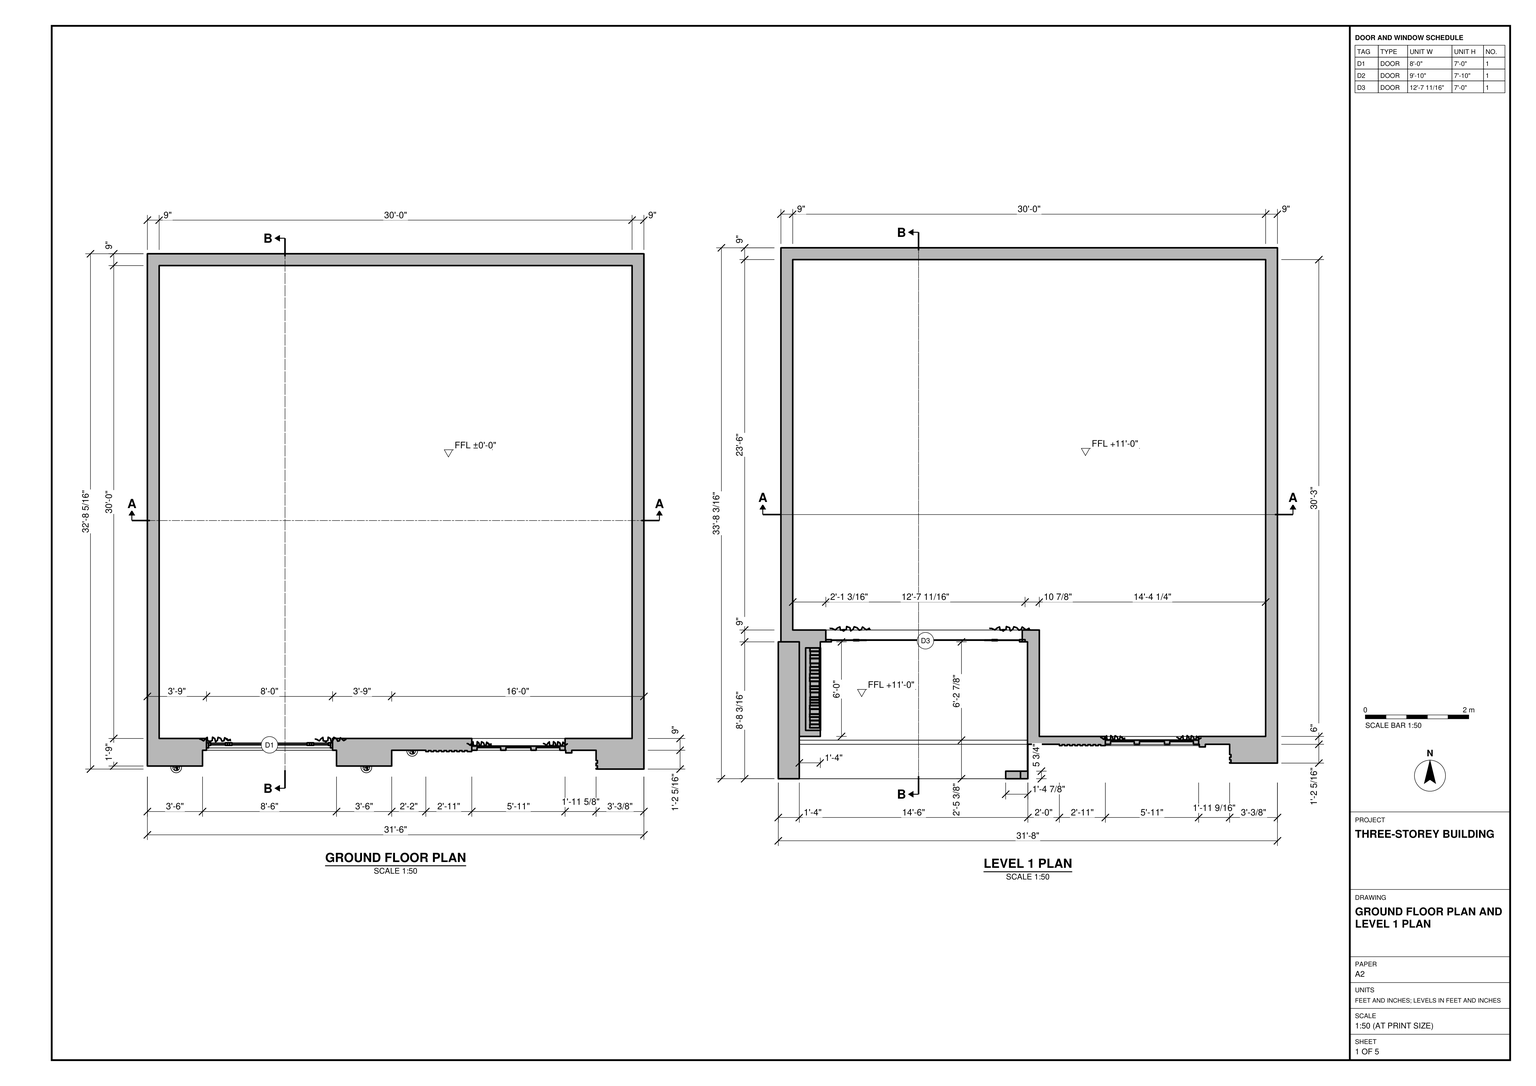
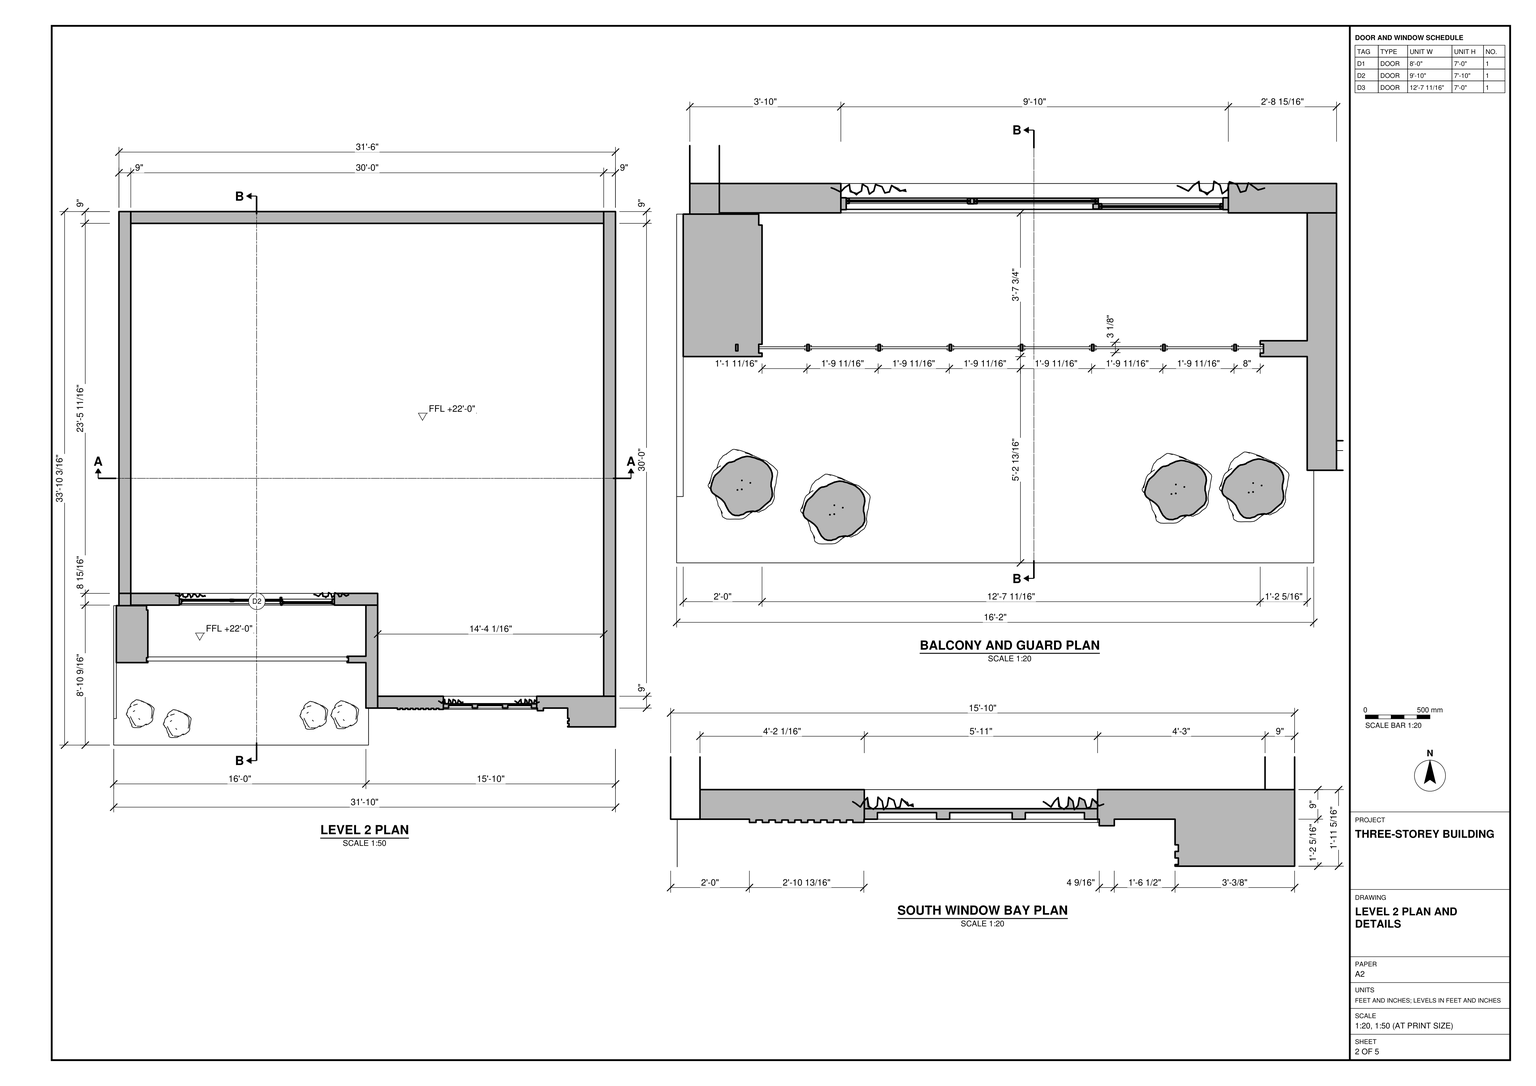
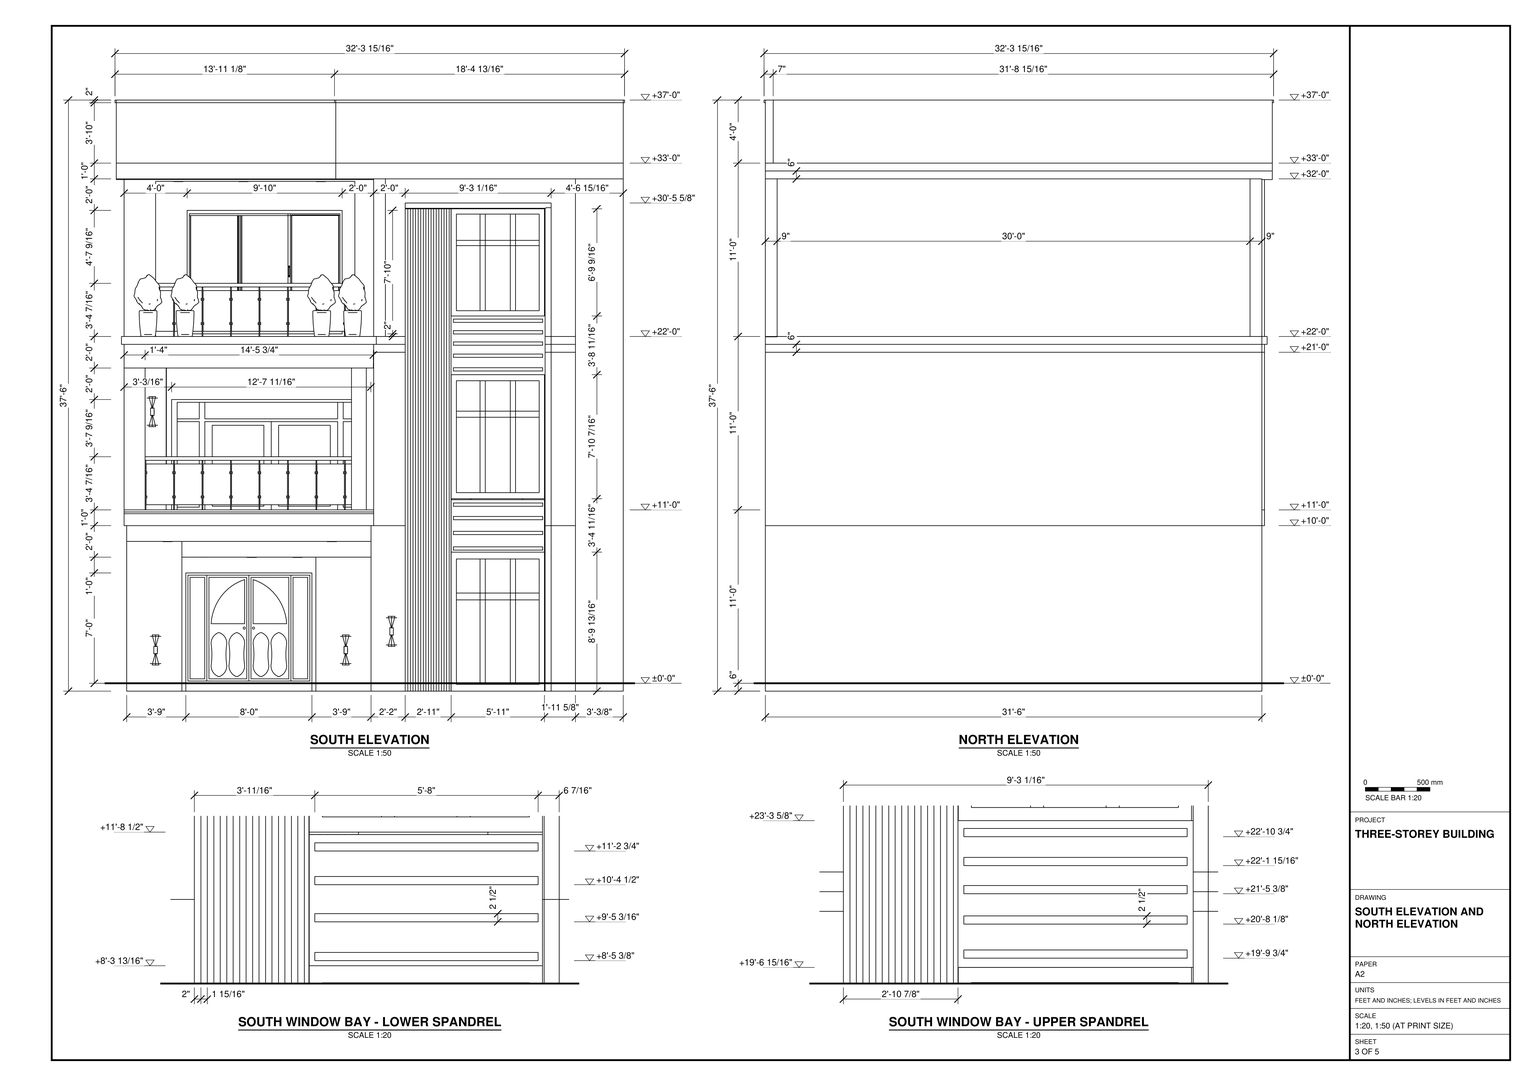
Build the three-storey building in SketchUp from task_files/diagram_01.pdf. Work in feet and inches. Orient the entrance to the south as drawn. The overall dimensions, including projections, are 32'-3 15/16" across the south elevation, 33'-10 3/16" from front to back and 37'-6" from base to top. Set the finished floor levels at ±0'-0", +11'-0" and +22'-0".

Use the floor plans to lay out the 9" perimeter walls and the changes in wall thickness and alignment at the south facade. Keep the main floor areas open as drawn. Model the base, floor slabs and flat roof with its parapet. On the left of the south elevation, place the double entrance with sidelights below the two balconies. Set the balcony doors back behind the glass guards, and extend the upper balcony slab beyond its guard as shown in the balcony plan. On the right, align the divided windows vertically. Model the ribbed strip beside the glazing and the horizontal bands between windows, using the enlarged spandrel details. Keep the north elevation plain apart from the slab and roof lines.

Place the potted plants on the upper balcony and wall lights where drawn. Decor and loose items may be any suitable library components. Keep shell elements such as walls, slabs and roof, and each furniture or joinery piece, in separate groups or components; use components for repeated parts. Save one SketchUp model as output_files/three_storey_building_with_balconies_and_window_bay.skp.

# SketchUp Ruby script. Lengths in inches.
U = 1.inch
M = Sketchup.active_model
def pt(a) = Geom::Point3d.new(a.map { |v| v * U })
def face(e, loops, mat)
  f = e.add_face(loops[0].map { |a| pt(a) })
  loops[1..].each { |l| e.add_face(l.map { |a| pt(a) }).erase! }
  f.material = f.back_material = mat if mat
  f
end
# faces: each face lists its corners as indices into pts; further lists are holes
def faces(e, pts, list, mat = nil) = list.each { |f| face(e, (f[0].is_a?(Array) ? f : [f]).map { |l| l.map { |i| pts[i] } }, mat) }
# xy, xz, yz: faces in a plane at the given z, y or x. An outline is a flat list of corners, or four numbers for a rectangle; further outlines are holes
def ring(l) = l.size == 4 ? [[l[0], l[1]], [l[2], l[1]], [l[2], l[3]], [l[0], l[3]]] : l.each_slice(2).to_a
def flat(e, list, mat, &to3) = list.each { |f| face(e, (f[0].is_a?(Array) ? f : [f]).map { |l| ring(l).map { |u, v| to3.(u, v) } }, mat) }
def xy(e, z, list, mat = nil) = flat(e, list, mat) { |x, y| [x, y, z] }
def xz(e, y, list, mat = nil) = flat(e, list, mat) { |x, z| [x, y, z] }
def yz(e, x, list, mat = nil) = flat(e, list, mat) { |y, z| [x, y, z] }
def lines(e, pts, list) = list.each { |a, b| e.add_line(pt(pts[a]), pt(pts[b])) }
# prism: a flat outline (further loops are holes) pulled along v
def prism(e, loops, v, mat = nil)
  f = face(e, loops, mat); d = Geom::Vector3d.new(v.map { |x| x * U })
  f.pushpull(f.normal.samedirection?(d) ? d.length : -d.length)
end
def box(e, o, s, mat = nil) = prism(e, [[o, [o[0] + s[0], o[1], o[2]], [o[0] + s[0], o[1] + s[1], o[2]], [o[0], o[1] + s[1], o[2]]]], [0, 0, s[2]], mat)
def at(x, y, z, deg = 0) = Geom::Transformation.translation(pt([x, y, z])) * Geom::Transformation.rotation(ORIGIN, Z_AXIS, deg.degrees)
def axes(o, x, y, z) = Geom::Transformation.new([*x, 0, *y, 0, *z, 0, *pt(o).to_a, 1])
def part(name) = M.definitions.add(name)
# library, detail: a bought-in or finely detailed component or shape, given as its bounding box
def library(name, o, s) = part(name).tap { |d| box(d.entities, o, s) }
def detail(e, o, s) = box(e.add_group.entities, o, s)
def put(e, d, t, mat = nil) = e.add_instance(d, t).tap { |i| i.material = mat if mat }
def group(e, t, mat = nil) = e.add_group.tap { |g| g.transformation = t; g.material = mat if mat }.entities
root = M.entities
M.materials.add("Emissive").color = [231, 236, 189]
M.materials["Emissive"].alpha = 1
M.materials.add("Glass Window Turquoise Blue").color = [210, 210, 210]
M.materials["Glass Window Turquoise Blue"].alpha = 0.25
M.materials.add("[0131_Silver]").color = [28, 28, 28]
M.materials.add("[Color A08]").color = [102, 0, 0]
M.materials.add("[Color M06]").color = [86, 86, 86]
M.materials.add("[Color M07]").color = [58, 58, 58]
M.materials.add("[Translucent_Glass_Blue]1").color = [255, 255, 255]
M.materials["[Translucent_Glass_Blue]1"].alpha = 0
M.materials.add("[Wood Cherry Original]").color = [152, 86, 42]
c1 = library("storefront door with transom",[0.96,31.97,0],[7.26,76.03,84.48])
c2 = library("Double Doors",[0,0,0],[118.11,4.72,98.43])
c3 = library("Sliding-door-2700x2100x89",[-27.94,-98.64,-16.57],[106.3,5.83,82.68])
c4 = library("Curtains 004",[-15.59,-2.26,0],[31.18,4.52,116.91])
c5 = library("Books  43-02",[-15.21,-3.875,0],[30.42,7.76,10.71])
c6 = library("Books and Flasks 103-12",[-7.1,-3.71,0],[14.22,7.42,6.38])
c7 = part("Group\#11")
xy(c7.entities,0,[[0,0,0.39,2.125]],"[0131_Silver]")
xy(c7.entities,1.5,[[0,0,0.39,2.125]],"[0131_Silver]")
xz(c7.entities,0,[[0,0,0.39,1.5]],"[0131_Silver]")
xz(c7.entities,2.125,[[0,0,0.39,1.5]],"[0131_Silver]")
yz(c7.entities,0,[[0,0,2.125,1.5]],"[0131_Silver]")
yz(c7.entities,0.39,[[0,0,2.125,1.5]],"[0131_Silver]")
c8 = part("Glass railing panel")
xy(c8.entities,0,[[-0.59,0,0,63.98]])
xy(c8.entities,37.71,[[-0.59,0,0,63.98]])
xz(c8.entities,0,[[-0.59,0,0,37.71]])
xz(c8.entities,63.98,[[-0.59,0,0,37.71]])
yz(c8.entities,-0.59,[[0,0,63.98,37.71]])
yz(c8.entities,0,[[0,0,63.98,0,63.98,37.71,0,37.71,0,30.53,1.75,30.53,1.75,28.71,0,28.71],[-0.4,28.71,0,30.53],[0,28.71,1.75,30.53]])
p = [[0,63.98,30.53],[0.39,63.98,30.53]]
lines(c8.entities,p,[[0,1]])
put(c8.entities,c7,axes([0,62.22,28.71],[1,0,0],[0,1.01246,0],[0,0,1.2158]))
put(c8.entities,c7,axes([0,62.22,6.27],[1,0,0],[0,1.01246,0],[0,0,1.2158]))
put(c8.entities,c7,axes([0,0.6,28.71],[1,0,0],[0,1.01246,0],[0,0,1.2158]))
put(c8.entities,c7,axes([0,0.6,6.27],[1,0,0],[0,1.01246,0],[0,0,1.2158]))
put(c8.entities,c7,axes([-0.98,0.6,28.71],[1,0,0],[0,1.01246,0],[0,0,1.2158]))
put(c8.entities,c7,axes([-0.98,62.22,6.27],[1,0,0],[0,1.01246,0],[0,0,1.2158]))
put(c8.entities,c7,axes([-0.98,0.6,6.27],[1,0,0],[0,1.01246,0],[0,0,1.2158]))
put(c8.entities,c7,axes([-0.98,62.22,28.71],[1,0,0],[0,1.01246,0],[0,0,1.2158]))
c9 = part("Group\#2")
xz(c9.entities,0,[[0,0,1.97,38.58]])
xz(c9.entities,1.97,[[0,0,1.97,38.58]])
yz(c9.entities,0,[[0,0,1.97,37.71]])
yz(c9.entities,1.97,[[0,0,1.97,37.71]])
c10 = part("Glass balcony railing")
xy(c10.entities,37.71,[[2.51,0,3.15,0.39,3.15,0]])
xy(c10.entities,37.71,[[0,0,0.54,520.67],[2.51,0,2.51,63.58,3.15,0.39],[3.15,0.39,2.51,63.58,2.51,520.67,3.15,520.67]],"[0131_Silver]")
xy(c10.entities,38.58,[[0.54,496.0625,2.51,520.67]])
xy(c10.entities,38.58,[[0.54,0,2.51,496.0625]],"[0131_Silver]")
xy(c10.entities,40.46,[[0,0,3.15,520.67]],"[0131_Silver]")
xz(c10.entities,0,[[0,37.71,0.54,37.71,0.54,38.58,2.51,38.58,2.51,37.71,3.15,37.71,3.15,40.46,0,40.46]],"[0131_Silver]")
xz(c10.entities,520.67,[[0,37.71,0,40.46,3.15,40.46,3.15,37.71,2.51,37.71,2.51,38.58,0.54,38.58,0.54,37.71]])
yz(c10.entities,0,[[0,37.71,520.67,40.46]],"[0131_Silver]")
yz(c10.entities,0.54,[[496.0625,37.71,520.67,38.58]])
yz(c10.entities,0.54,[[0,37.71,496.0625,38.58]],"[0131_Silver]")
yz(c10.entities,2.51,[[0,37.71,496.0625,38.58],[496.0625,37.71,520.67,38.58]])
yz(c10.entities,3.15,[[0,37.71,520.67,40.46]],"[0131_Silver]")
put(c10.entities,c8,axes([1.8,65.35,3.9375],[1,0,0],[0,0.98769,0],[0,0,0.8225]),"[Translucent_Glass_Blue]1")
put(c10.entities,c8,axes([1.8,130.31,3.9375],[1,0,0],[0,0.98769,0],[0,0,0.8225]),"[Translucent_Glass_Blue]1")
put(c10.entities,c8,axes([1.8,195.28,3.9375],[1,0,0],[0,0.98769,0],[0,0,0.8225]),"[Translucent_Glass_Blue]1")
put(c10.entities,c8,axes([1.8,260.24,3.9375],[1,0,0],[0,0.98769,0],[0,0,0.8225]),"[Translucent_Glass_Blue]1")
put(c10.entities,c8,axes([1.8,325.2,3.9375],[1,0,0],[0,0.98769,0],[0,0,0.8225]),"[Translucent_Glass_Blue]1")
put(c10.entities,c8,axes([1.8,390.16,3.9375],[1,0,0],[0,0.98769,0],[0,0,0.8225]),"[Translucent_Glass_Blue]1")
put(c10.entities,c8,axes([1.8,455.12,3.9375],[1,0,0],[0,0.98769,0],[0,0,0.8225]),"[Translucent_Glass_Blue]1")
put(c10.entities,c8,axes([1.8,0.39,3.9375],[1,0,0],[0,0.98769,0],[0,0,0.8225]),"[Translucent_Glass_Blue]1")
put(c10.entities,c9,at(0.54,128.9375,0),"[0131_Silver]")
g1 = group(c10.entities,at(0.54,63.98,0),"[0131_Silver]")
xz(g1,0,[[0,0,1.97,38.58]])
xz(g1,1.97,[[0,0,1.97,38.58]])
yz(g1,0,[[0,0,1.97,37.71]])
yz(g1,1.97,[[0,0,1.97,37.71]])
put(c10.entities,c9,at(0.54,193.9,0),"[0131_Silver]")
put(c10.entities,c9,at(0.54,258.86,0),"[0131_Silver]")
put(c10.entities,c9,at(0.54,323.82,0),"[0131_Silver]")
put(c10.entities,c9,at(0.54,388.78,0),"[0131_Silver]")
put(c10.entities,c9,at(0.54,453.74,0),"[0131_Silver]")
put(c10.entities,c9,at(0.54,518.7,0),"[0131_Silver]")
c11 = part("Glass+Railing")
put(c11.entities,c10,axes([0,0,0],[1,0,0],[0,0.95652,0],[0,0,1]),"[0131_Silver]")
c12 = library("Tlon Light 650 Ceiling 152 007",[-12.8,-12.8,-3.78],[25.6,25.6,3.58])
c13 = library("Omni Light",[-12,-12,-12],[24,24,24])
c14 = library("Wall Light 02",[-3.77,-223.45,-4.0625],[223.9,240.38,31.25])
c15 = library("Potted Plant 60-25",[-10.7,-10.47,0],[21.2,21.27,47.12])
c16 = part("Group\#1")
xy(c16.entities,0,[[0,0,71.03,3.2]],"[Color M07]")
xy(c16.entities,4,[[4,0,22,2],[26,0,45.03,2],[49.03,0,67.03,2]],"[Color M07]")
xy(c16.entities,53.5625,[[49.03,0,67.03,2]],"[Color A08]")
xy(c16.entities,53.5625,[[4,0,22,2],[26,0,45.03,2]],"[Color M07]")
xy(c16.entities,57.5625,[[4,0,22,2],[26,0,45.03,2],[49.03,0,67.03,2]],"[Color M07]")
xy(c16.entities,77.5625,[[4,0,22,2],[26,0,45.03,2],[49.03,0,67.03,2]],"[Color M07]")
xy(c16.entities,81.5625,[[0,0,71.03,3.2]],"[Color M07]")
xz(c16.entities,0,[[[0,0,71.03,81.5625],[4,4,67.03,77.5625]],[22,4,26,53.5625],[45.03,4,49.03,53.5625],[4,53.5625,22,57.5625],[22,53.5625,26,57.5625],
  [26,53.5625,45.03,57.5625],[45.03,53.5625,49.03,57.5625],[49.03,53.5625,67.03,57.5625],[22,57.5625,26,77.5625],[45.03,57.5625,49.03,77.5625]],"[Color M07]")
xz(c16.entities,2,[[4,4,22,53.5625],[26,4,45.03,53.5625],[49.03,4,67.03,53.5625],[4,57.5625,22,77.5625],[26,57.5625,45.03,77.5625],
  [49.03,57.5625,67.03,77.5625]],"Glass Window Turquoise Blue")
xz(c16.entities,3.2,[[0,0,71.03,81.5625]],"Glass Window Turquoise Blue")
yz(c16.entities,0,[[0,0,3.2,81.5625]],"[Color M07]")
yz(c16.entities,4,[[0,4,2,53.5625],[0,57.5625,2,77.5625]],"[Color M07]")
yz(c16.entities,22,[[0,4,2,53.5625],[0,57.5625,2,77.5625]],"[Color M07]")
yz(c16.entities,26,[[0,4,2,53.5625],[0,57.5625,2,77.5625]],"[Color M07]")
yz(c16.entities,45.03,[[0,4,2,53.5625],[0,57.5625,2,77.5625]],"[Color M07]")
yz(c16.entities,49.03,[[0,57.5625,2,77.5625]],"[Color A08]")
yz(c16.entities,49.03,[[0,4,2,53.5625]],"[Color M07]")
yz(c16.entities,67.03,[[0,4,2,53.5625],[0,57.5625,2,77.5625]],"[Color M07]")
yz(c16.entities,71.03,[[0,0,3.2,81.5625]],"[Color M07]")
xy(root,0,[[350.54,13.89,350.54,14.39,351.54,14.39,351.54,16.39,350.54,16.39,350.54,18.39,351.54,18.39,351.54,20.39,350.54,20.39,350.54,28.2,332.03,28.2,332.03,26.2,327.45,26.2,327.45,28.2,326.9375,28.2,326.9375,37.2,377.9375,37.2,377.9375,397.2,17.9375,397.2,17.9375,37.2,53.9375,37.2,53.9375,28.2,50.9375,28.2,50.9375,16.2,8.9375,16.2,8.9375,406.2,386.9375,406.2,386.9375,13.89],[152.9375,16.2,152.9375,28.2,149.9375,28.2,149.9375,37.2,255.91,37.2,255.91,28.2,255.82,28.2,255.82,27.2,252.4375,27.2,252.4375,27.95,250.5,27.95,250.5,27.2,248.5,27.2,248.5,27.95,246.56,27.95,246.56,27.2,244.5625,27.2,244.5625,27.95,242.62,27.95,242.62,27.2,240.625,27.2,240.625,27.95,238.68,27.95,238.68,27.2,236.6875,27.2,236.6875,27.95,234.75,27.95,234.75,27.2,232.75,27.2,232.75,27.95,230.81,27.95,230.81,27.2,228.8125,27.2,228.8125,27.95,226.87,27.95,226.87,27.2,224.875,27.2,224.875,27.95,222.93,27.95,222.93,27.2,220.9375,27.2,220.9375,28.2,194.9375,28.2,194.9375,16.2],[53.9375,28.2,53.9375,37.2,17.9375,37.2,17.9375,397.2,377.9375,397.2,377.9375,37.2,149.9375,37.2,149.9375,28.2],[255.91,28.2,326.9375,37.2]])
xy(root,6,[[53.9375,28.2,149.9375,28.2,149.9375,37.2,377.9375,37.2,377.9375,397.2,17.9375,397.2,17.9375,37.2,53.9375,37.2]])
xy(root,90,[[53.9375,28.2,149.9375,37.2]])
xy(root,102,[[50.9375,16.2,152.9375,28.2]])
xy(root,105.8125,[[255.91,27.2,326.9375,28.2],[255.91,28.2,255.91,37.2,325.93,37.2,326.9375,28.2]])
xy(root,107.37,[[257.61,27.2,325.61,28]])
xy(root,109.87,[[257.61,27.2,325.61,28]])
xy(root,114,[[8.9375,4.2,194.9375,16.2],[326.9375,28.2,325.93,37.2,326.9375,37.2]])
xy(root,119.18,[[257.61,27.2,325.61,28]])
xy(root,121.68,[[257.61,27.2,325.61,28]])
xy(root,126,[[6.9375,2.2,196.9375,4.2],[6.9375,4.2,8.9375,106.2],[194.9375,4.2,196.9375,28.2],[326.9375,28.2,325.93,34.2,326.9375,34.2],[255.91,34.2,325.93,37.2],
  [17.9375,37.2,377.9375,397.2]])
xy(root,130.49,[[257.61,27.2,325.61,28]])
xy(root,132.99,[[257.61,27.2,325.61,28]])
xy(root,135.12,[[6.9375,2.2,196.9375,3]])
xy(root,136.4,[[6.9375,2,196.9375,3]])
xy(root,138,[[6.9375,2,22.9375,106.2],[22.9375,2,180.05,2,180.05,7.76,196.66,7.76,196.66,106.2,192.66,106.2,192.66,115.2,43.125,115.2,43.125,106.2,38.9375,106.2,38.9375,34.2,22.9375,34.2],[180.05,2,191.33,7.76],[191.33,2,191.33,7.76,196.66,7.76,196.66,28.2,196.9375,28.2,196.9375,2],[205.66,34.2,377.9375,34.2,377.9375,397.2,17.9375,397.2,17.9375,115.2,205.66,115.2]])
xy(root,140.74,[[257.61,27.2,325.61,28]])
xy(root,142.58,[[38.9375,38.78,39.14,101.62]])
xy(root,142.58,[[27.75,38.78,38.9375,101.62]],"[Wood Cherry Original]")
xy(root,143.24,[[257.61,27.2,325.61,28]])
xy(root,145.75,[[255.91,27.2,326.9375,28.2],[255.91,28.2,326.9375,34.2]])
xy(root,174.74,[[27.75,38.78,29.75,101.62]],"Emissive")
xy(root,174.74,[[29.75,38.78,38.5625,101.62]],"[Wood Cherry Original]")
xy(root,177.44,[[27.75,38.78,38.5625,101.62]],"[Wood Cherry Original]")
xy(root,197.68,[[27.75,38.78,29.75,101.62]],"Emissive")
xy(root,197.68,[[29.75,38.78,38.5625,101.62]],"[Wood Cherry Original]")
xy(root,200.38,[[27.75,38.78,38.5625,101.62]],"[Wood Cherry Original]")
xy(root,220.61,[[27.75,38.78,29.75,101.62]],"Emissive")
xy(root,220.61,[[29.75,38.78,38.5625,101.62]],"[Wood Cherry Original]")
xy(root,222,[[43.125,106.2,192.66,115.2]])
xy(root,223.32,[[27.75,38.78,38.5625,101.62]],"[Wood Cherry Original]")
xy(root,240.93,[[255.91,28.2,326.9375,34.2]])
xy(root,240.94,[[255.82,27.2,327.45,28.2]])
xy(root,243.74,[[257.61,27.2,325.61,28]])
xy(root,246,[[6.9375,2,22.9375,2.2],[22.9375,2,22.9375,6.57,180.05,7.76,180.05,2],[180.05,2,191.33,2.2],[191.33,2,196.66,2.2]])
xy(root,246.24,[[257.61,27.2,325.61,28]])
xy(root,247.42,[[38.9375,38.78,39.14,101.62]])
xy(root,247.42,[[27.75,38.78,29.75,101.62]],"Emissive")
xy(root,247.42,[[29.75,38.78,38.9375,101.62]],"[Wood Cherry Original]")
xy(root,252,[[22.9375,6.57,23.04,34.2],[191.33,7.76,196.66,28.2]])
xy(root,252,[[23.04,6.57,23.04,34.2,38.9375,34.2,38.9375,106.2,196.66,106.2,196.66,28.2,191.33,28.2,191.33,7.76,180.05,7.76]],"[Wood Cherry Original]")
xy(root,254.12,[[257.61,27.2,325.61,28]])
xy(root,256.62,[[257.61,27.2,325.61,28]])
xy(root,258,[[196.9375,2.2,196.9375,28.2,196.66,28.2],[191.33,7.76,191.33,28.2,196.66,28.2],[205.66,34.2,205.66,115.2,17.9375,115.2,17.9375,397.2,377.9375,397.2,377.9375,34.2],[22.9375,34.2,38.9375,106.2],[196.66,34.2,205.66,115.2],
  [8.9375,106.2,17.9375,115.2],[17.9375,106.2,196.66,115.2],[8.9375,115.2,17.9375,397.2],[8.9375,397.2,377.9375,406.2]])
xy(root,263.37,[[257.61,27.2,325.61,28]])
xy(root,264,[[4.9375,0,4.9375,2.2,6.9375,2.2,6.9375,2,196.9375,2,196.9375,2.2,198.9375,2.2,198.9375,0],[4.9375,2.2,6.9375,106.2],[196.9375,2.2,198.9375,28.2]])
xy(root,265.87,[[257.61,27.2,325.61,28]])
xy(root,269.75,[[377.9375,37.21,386.9375,406.2]])
xy(root,270,[[4.9375,0,198.9375,0,198.9375,28.2,196.9375,28.2,196.9375,62.82,182.63,62.82,182.63,67.64,196.9375,67.64,196.9375,106.57,17.9375,106.57,17.9375,106.2,29.9375,106.2,29.9375,63.89,30.9375,63.89,30.9375,62.82,6.9375,62.82,6.9375,20.2,4.9375,20.2],[4.9375,20.2,6.9375,106.2],[196.9375,28.2,205.875,106.57],[377.9375,37.2,386.9375,37.21],[205.875,37.21,377.9375,37.21,377.9375,397.2,17.9375,397.2,17.9375,115.53,205.875,115.53],
  [377.9375,37.21,386.9375,406.2],[6.9375,62.82,6.9375,106.2,29.9375,106.2,29.9375,63.89,30.9375,63.89,30.9375,62.82],[8.9375,106.2,17.9375,106.57],[8.9375,106.57,17.9375,115.53],[17.9375,106.57,205.875,115.53],
  [54.9375,106.57,172.9375,107.04],[8.9375,115.53,17.9375,406.2],[17.9375,397.2,377.9375,406.2]])
xy(root,271.07,[[182.63,63.89,183.63,66.57]])
xy(root,271.93,[[257.61,27.2,325.61,28]])
xy(root,272,[[54.9375,106.57,172.9375,115.53]])
xy(root,272.74,[[29.9375,66.57,30.9375,102.87]])
xy(root,274.43,[[257.61,27.2,325.61,28]])
xy(root,280.74,[[257.61,27.2,325.61,28]])
xy(root,283.24,[[257.61,27.2,325.61,28]])
xy(root,285.625,[[255.82,27.2,326.9375,28.2],[326.9375,27.2,327.45,28.2],[255.91,28.2,326.9375,37.21]])
xy(root,366,[[54.9375,106.57,172.9375,115.53]])
xy(root,367.1875,[[220.9375,27.2,222.93,27.2,222.93,27.95,224.875,27.95,224.875,27.2,226.87,27.2,226.87,27.95,228.8125,27.95,228.8125,27.2,230.81,27.2,230.81,27.95,232.75,27.95,232.75,27.2,234.75,27.2,234.75,27.95,236.6875,27.95,236.6875,27.2,238.68,27.2,238.68,27.95,240.625,27.95,240.625,27.2,242.62,27.2,242.62,27.95,244.5625,27.95,244.5625,27.2,246.56,27.2,246.56,27.95,248.5,27.95,248.5,27.2,250.5,27.2,250.5,27.95,252.4375,27.95,252.4375,27.2,255.82,27.2,255.82,28.2,220.9375,28.2],[255.91,28.2,326.9375,37.21]])
xy(root,367.63,[[220.9375,26.2,327.45,28.2]])
xy(root,371.63,[[220.9375,26.2,332.03,28.2]])
xy(root,385.6,[[29.9375,66.57,30.9375,102.87]])
xy(root,388.0625,[[30.9375,62.82,182.63,63.89],[29.9375,66.57,182.63,67.64],[30.9375,67.64,30.9375,106.2,17.9375,106.2,17.9375,106.57,196.9375,106.57,196.9375,67.64],[29.9375,67.64,30.9375,106.2]])
xy(root,389.0625,[[29.9375,63.89,183.63,66.57]],"Emissive")
xy(root,389.4375,[[[1,56.44,196.9375,62.82],[2.75,57.69,194.75,59.94]],[1,62.82,6.9375,106.2],[30.9375,62.82,196.9375,67.64],[1,106.2,8.9375,106.57],[1,106.57,8.9375,115.53],
  [1,115.53,8.9375,406.2]])
xy(root,390,[[168.1,13.89,168.1,45.51,1,45.51,1,56.44,196.9375,56.44,196.9375,28.2,350.54,28.2,350.54,20.39,174.6,20.39,174.6,52,3.64,52,3.64,50,172.6,50,172.6,46,170.6,46,170.6,48,3.64,48,3.64,46,168.6,46,168.6,14.39,350.54,14.39,350.54,13.89],[350.54,13.89,377.9375,13.89,377.9375,37.21,205.875,37.21,205.875,28.2,350.54,28.2,350.54,20.39,351.54,20.39,351.54,18.39,350.54,18.39,350.54,16.39,351.54,16.39,351.54,14.39,350.54,14.39],[377.9375,13.89,386.9375,37.2],[170.6,16.39,170.6,46,172.6,46,172.6,18.39,350.54,18.39,350.54,16.39],[196.9375,28.2,205.875,106.57],
  [377.9375,37.2,386.9375,37.21],[205.875,37.21,205.875,115.53,17.9375,115.53,17.9375,397.2,377.9375,397.2,377.9375,37.21],[377.9375,37.21,386.9375,406.2],[6.9375,62.82,17.9375,106.2],[17.9375,62.82,30.9375,106.2],
  [8.9375,106.2,17.9375,106.57],[8.9375,106.57,17.9375,115.53],[17.9375,106.57,54.9375,115.53],[54.9375,106.57,205.875,115.53],[8.9375,115.53,17.9375,406.2],
  [17.9375,397.2,377.9375,406.2]])
xy(root,390,[[350.54,14.39,351.54,16.39],[350.54,18.39,351.54,20.39]],"Emissive")
xy(root,390.4375,[[2.75,57.69,194.75,59.94]],"Emissive")
xy(root,391,[[168.6,14.39,168.6,46,170.6,46,170.6,16.39,350.54,16.39,350.54,14.39],[172.6,18.39,350.54,20.39],[172.6,20.39,174.6,46],[3.64,46,170.6,48],[172.6,46,174.6,52],
  [3.64,50,172.6,52]],"Emissive")
xy(root,402,[[168.1,13.89,174.1,51.51],[174.1,13.89,386.9375,19.89],[174.1,19.89,380.9375,19.89,380.9375,400.2,7,400.2,7,51.51,174.1,51.51],[380.9375,19.89,386.9375,406.2],[1,45.51,7,400.2],
  [7,45.51,168.1,51.51],[1,400.2,380.9375,406.2]])
xy(root,448,[[167.1,12.89,168.1,13.89],[168.1,12.89,386.9375,13.89],[386.9375,12.89,387.9375,13.89],[167.1,13.89,168.1,45.51],[386.9375,13.89,387.9375,406.2],
  [0,44.51,1,45.51],[1,44.51,167.1,45.51],[0,45.51,1,400.2]])
xy(root,450,[[167.1,12.89,168.1,13.89],[168.1,12.89,386.9375,13.89],[386.9375,12.89,387.9375,13.89],[167.1,13.89,168.1,45.51],[168.1,13.89,386.9375,13.89,386.9375,406.2,380.9375,406.2,380.9375,19.89,174.1,19.89,174.1,51.51,168.1,51.51],
  [386.9375,13.89,387.9375,406.2],[0,44.51,1,45.51],[1,44.51,167.1,45.51],[0,45.51,1,400.2],[1,45.51,168.1,45.51,168.1,51.51,7,51.51,7,400.2,1,400.2],
  [1,400.2,380.9375,406.2]])
xz(root,0,[[4.9375,264,198.9375,270]])
xz(root,2,[[6.9375,136.4,196.9375,138],[6.9375,138,22.9375,246],[180.05,138,191.33,246],[191.33,138,196.9375,138,196.9375,258,196.66,246,191.33,246],[6.9375,246,196.66,246,196.9375,258,196.9375,264,6.9375,264]])
xz(root,2.2,[[6.9375,126,196.9375,135.12]])
xz(root,3,[[6.9375,135.12,196.9375,136.4]])
xz(root,4.2,[[8.9375,114,194.9375,126]])
xz(root,6.57,[[22.9375,246.5,23.04,252]])
xz(root,7.76,[[180.05,138,191.33,252],[191.33,138,196.66,252],[180.05,252,191.33,258]])
xz(root,12.89,[[167.1,448,168.1,450],[168.1,448,386.9375,450],[386.9375,448,387.9375,450]])
xz(root,13.89,[[350.54,0,386.9375,390],[168.1,390,386.9375,402],[168.1,402,386.9375,448],[167.1,448,168.1,450],[168.1,448,386.9375,450],
  [386.9375,448,387.9375,450]])
xz(root,14.39,[[350.54,0,351.54,390],[168.6,390,170.6,391],[170.6,390,350.54,391]],"Emissive")
xz(root,16.2,[[8.9375,0,50.9375,114],[152.9375,0,194.9375,102],[50.9375,102,194.9375,114]])
xz(root,16.39,[[350.54,0,351.54,390],[170.6,390,350.54,391]],"Emissive")
xz(root,18.39,[[350.54,0,351.54,390],[172.6,390,350.54,391]],"Emissive")
xz(root,19.89,[[174.1,402,380.9375,450]])
xz(root,20.39,[[350.54,0,351.54,390],[174.6,390,350.54,391]],"Emissive")
xz(root,26.2,[[327.45,0,332.03,126],[327.45,126,332.03,258],[327.45,258,332.03,264],[327.45,264,332.03,270],[327.45,270,332.03,270,332.03,368.07,328.07,368.07,328.07,367.63,327.45,367.63],
  [220.9375,367.63,328.07,367.63,328.07,368.07,332.03,368.07,332.03,371.63,220.9375,371.63]])
xz(root,27.2,[[220.9375,0,222.93,367.1875],[224.875,0,226.87,367.1875],[228.8125,0,230.81,367.1875],[232.75,0,234.75,367.1875],[236.6875,0,238.68,367.1875],
  [240.625,0,242.62,367.1875],[244.5625,0,246.56,367.1875],[248.5,0,250.5,367.1875],[252.4375,0,254.43,367.1875],[254.43,0,255.82,367.1875],
  [[255.91,105.8125,326.9375,145.75],[257.61,140.74,325.61,143.24],[257.61,130.49,325.61,132.99],[257.61,119.18,325.61,121.68],[257.61,107.37,325.61,109.87]],[[255.82,240.94,327.45,285.625],[257.61,280.74,325.61,283.24],[257.61,271.93,325.61,274.43],[257.61,263.37,325.61,265.87],[257.61,254.12,325.61,256.62],[257.61,243.74,325.61,246.24]]])
xz(root,27.95,[[222.93,0,224.875,367.1875],[226.87,0,228.8125,367.1875],[230.81,0,232.75,367.1875],[234.75,0,236.6875,367.1875],[238.68,0,240.625,367.1875],
  [242.62,0,244.5625,367.1875],[246.56,0,248.5,367.1875],[250.5,0,252.4375,367.1875]])
xz(root,28,[[257.61,107.37,325.61,109.87],[257.61,119.18,325.61,121.68],[257.61,130.49,325.61,132.99],[257.61,140.74,325.61,143.24],[257.61,243.74,325.61,246.24],
  [257.61,254.12,325.61,256.62],[257.61,263.37,325.61,265.87],[257.61,271.93,325.61,274.43],[257.61,280.74,325.61,283.24]])
xz(root,28.2,[[50.9375,0,53.9375,0,53.9375,90,149.9375,90,149.9375,0,152.9375,0,152.9375,102,50.9375,102],[53.9375,0,149.9375,6],[194.9375,0,220.9375,126],[255.82,0,255.91,126],[326.9375,0,327.45,126],
  [332.03,0,350.54,126],[255.91,105.8125,326.9375,145.75],[196.9375,126,220.9375,258],[255.82,126,255.91,126,255.91,240.93,326.9375,240.93,326.9375,126,327.45,126,327.45,240.94,255.82,240.94],[332.03,126,350.54,258],
  [196.66,138,196.9375,258],[191.33,252,196.66,258],[196.9375,258,220.9375,264],[332.03,258,350.54,264],[198.9375,264,220.9375,270],
  [332.03,264,350.54,270],[196.9375,270,205.875,390],[205.875,270,220.9375,270,220.9375,367.1875,326.9375,367.1875,326.9375,285.625,327.45,285.625,327.45,367.63,220.9375,367.63,220.9375,371.63,332.03,371.63,332.03,270,350.54,270,350.54,390,205.875,390],[255.82,285.625,255.91,367.1875]])
xz(root,34.2,[[255.91,126,326.9375,138],[22.9375,138,38.9375,138,38.9375,252,23.04,252,23.04,249.69,22.9375,249.69],[205.66,138,205.66,258,377.9375,258,377.9375,138,326.9375,138,326.9375,240.93,255.91,240.93,255.91,138],[255.91,138,326.9375,145.75],[22.9375,249.69,23.04,252],
  [22.9375,252,38.9375,258]])
xz(root,37.2,[[17.9375,0,53.9375,6],[149.9375,0,255.91,6],[255.91,0,326.9375,6],[326.9375,0,377.9375,6],[17.9375,6,17.9375,126,255.91,126,255.91,6,149.9375,6,149.9375,90,53.9375,90,53.9375,6],
  [326.9375,6,326.9375,114,325.93,114,325.93,126,377.9375,126,377.9375,6],[255.91,105.8125,325.93,126],[377.9375,270,386.9375,390]])
xz(root,37.21,[[377.9375,269.75,386.9375,270],[[205.875,270,377.9375,390],[255.91,285.625,326.9375,367.1875]],[377.9375,270,386.9375,390]])
xz(root,38.78,[[38.9375,142.58,39.14,247.42]],"Glass Window Turquoise Blue")
xz(root,38.78,[[27.75,142.58,27.75,174.74,38.5625,174.74,38.5625,177.44,27.75,177.44,27.75,197.68,38.5625,197.68,38.5625,200.38,27.75,200.38,27.75,220.61,38.5625,220.61,38.5625,223.32,27.75,223.32,27.75,247.42,38.9375,247.42,38.9375,142.58]],"[Wood Cherry Original]")
xz(root,44.51,[[0,448,1,450],[1,448,167.1,450]])
xz(root,45.51,[[1,390,168.1,402],[1,402,168.1,448],[0,448,1,450],[1,448,167.1,450],[167.1,448,168.1,450]])
xz(root,46,[[3.64,390,168.6,391]],"Emissive")
xz(root,48,[[3.64,390,170.6,391]],"Emissive")
xz(root,50,[[3.64,390,172.6,391]],"Emissive")
xz(root,51.51,[[7,402,168.1,450],[168.1,402,174.1,450]])
xz(root,52,[[3.64,390,172.6,391],[172.6,390,174.6,391]],"Emissive")
xz(root,56.44,[[1,389.4375,196.9375,390]])
xz(root,57.69,[[2.75,389.4375,194.75,390.4375]],"Emissive")
xz(root,59.94,[[2.75,389.4375,194.75,390.4375]],"Emissive")
xz(root,62.82,[[6.9375,270,30.9375,270,30.9375,388.0625,182.63,388.0625,182.63,270,196.9375,270,196.9375,389.4375,6.9375,389.4375],[6.9375,389.4375,17.9375,390],[17.9375,389.4375,30.9375,390]])
xz(root,63.89,[[29.9375,270,30.9375,272.74],[29.9375,272.74,30.9375,389.0625]])
xz(root,63.89,[[182.63,271.07,183.63,388.0625],[30.9375,388.0625,183.63,389.0625]],"Emissive")
xz(root,66.57,[[29.9375,272.74,30.9375,385.6]])
xz(root,66.57,[[182.63,271.07,183.63,388.0625],[29.9375,388.0625,183.63,389.0625]],"Emissive")
xz(root,67.64,[[182.63,270,196.9375,388.0625],[30.9375,388.0625,196.9375,389.4375]])
xz(root,101.62,[[38.9375,142.58,39.14,247.42]])
xz(root,101.62,[[27.75,142.58,38.9375,142.58,38.9375,247.42,27.75,247.42,27.75,223.32,38.5625,223.32,38.5625,220.61,27.75,220.61,27.75,200.38,38.5625,200.38,38.5625,197.68,27.75,197.68,27.75,177.44,38.5625,177.44,38.5625,174.74,27.75,174.74]],"[Wood Cherry Original]")
xz(root,102.87,[[29.9375,272.74,30.9375,385.6]])
xz(root,106.2,[[6.9375,126,8.9375,138],[6.9375,138,8.9375,258],[8.9375,138,17.9375,258],[17.9375,138,22.9375,258],[38.9375,138,43.125,138,43.125,222,192.66,222,192.66,138,196.66,138,196.66,252,38.9375,252],
  [38.9375,252,196.66,258],[6.9375,258,8.9375,264],[4.9375,264,8.9375,270],[6.9375,270,8.9375,389.4375],[8.9375,270,17.9375,390],
  [17.9375,270,29.9375,388.0625],[17.9375,388.0625,30.9375,390],[6.9375,389.4375,8.9375,390]])
xz(root,106.57,[[[17.9375,270,196.9375,388.0625],[54.9375,272,172.9375,366]],[196.9375,270,205.875,390],[17.9375,388.0625,54.9375,390],[54.9375,388.0625,196.9375,390]])
xz(root,115.2,[[17.9375,138,17.9375,258,196.66,258,196.66,138,192.66,138,192.66,222,43.125,222,43.125,138],[196.66,138,205.66,258]])
xz(root,115.53,[[8.9375,270,17.9375,390],[[17.9375,270,205.875,390],[54.9375,272,172.9375,366]]])
xz(root,397.2,[[17.9375,0,377.9375,6],[17.9375,6,377.9375,126],[17.9375,138,377.9375,258],[17.9375,270,377.9375,390]])
xz(root,400.2,[[1,402,7,450],[7,402,380.9375,450],[0,448,1,450]])
xz(root,406.2,[[8.9375,0,386.9375,126],[8.9375,126,386.9375,258],[8.9375,258,386.9375,264],[8.9375,264,8.9375,270,377.9375,270,377.9375,269.75,386.9375,269.75,386.9375,264],[377.9375,269.75,386.9375,270],
  [8.9375,270,17.9375,390],[17.9375,270,377.9375,390],[377.9375,270,386.9375,390],[1,389.4375,1,396,386.9375,396,386.9375,390,8.9375,390,8.9375,389.4375],[1,396,386.9375,402],
  [1,402,380.9375,450],[380.9375,402,386.9375,450],[386.9375,448,387.9375,450]])
yz(root,0,[[44.51,448,45.51,450],[45.51,448,400.2,450]])
yz(root,1,[[56.44,389.4375,56.44,390,45.51,390,45.51,402,406.2,402,406.2,389.4375],[45.51,402,400.2,448],[400.2,402,406.2,450],[44.51,448,45.51,450],[45.51,448,400.2,450]])
yz(root,2.75,[[57.69,389.4375,59.94,390.4375]],"Emissive")
yz(root,3.64,[[46,390,48,391],[50,390,52,391]],"Emissive")
yz(root,4.9375,[[0,264,106.2,270]])
yz(root,6.9375,[[2.2,126,2.2,135.12,3,135.12,3,136.4,2,136.4,2,138,106.2,138,106.2,126],[2,138,2,246,2.2,246,106.2,258,106.2,138],[2,246,2,264,106.2,264,106.2,258,2.2,246],[62.82,270,106.2,389.4375],[62.82,389.4375,106.2,390]])
yz(root,7,[[51.51,402,400.2,450]])
yz(root,8.9375,[[16.2,0,16.2,114,4.2,114,4.2,126,406.2,126,406.2,0],[106.2,126,406.2,258],[106.2,258,406.2,264],[106.2,264,406.2,270],[106.2,270,106.57,389.4375],
  [106.57,270,115.53,389.4375],[115.53,270,406.2,389.4375],[106.2,389.4375,106.57,390],[106.57,389.4375,115.53,390],[115.53,389.4375,406.2,390]])
yz(root,17.9375,[[37.2,0,397.2,6],[37.2,6,397.2,126],[115.2,138,397.2,258],[106.2,270,106.57,388.0625],[106.57,270,115.53,390],
  [115.53,270,397.2,390],[397.2,270,406.2,390],[106.2,388.0625,106.57,390]])
yz(root,22.9375,[[2,138,34.2,138,34.2,249.69,6.57,246.5,6.57,246,2,246],[34.2,138,106.2,138,106.2,258,34.2,249.69],[2.2,246,6.57,246,6.57,246.5],[2.2,246,6.57,258,6.57,246.5],[6.57,246.5,6.57,252,34.2,252,34.2,249.69],
  [34.2,249.69,34.2,258,106.2,258],[6.57,252,34.2,258]])
yz(root,23.04,[[6.57,246.5,34.2,249.69,34.2,252,6.57,252]])
yz(root,27.75,[[38.78,142.58,101.62,174.74],[38.78,177.44,101.62,197.68],[38.78,200.38,101.62,220.61],[38.78,223.32,101.62,247.42]],"[Wood Cherry Original]")
yz(root,29.9375,[[63.89,270,66.57,272.74],[66.57,270,102.87,272.74],[102.87,270,106.2,385.6],[63.89,272.74,66.57,389.0625],[66.57,385.6,106.2,388.0625]],"Emissive")
yz(root,30.9375,[[62.82,270,63.89,388.0625],[66.57,272.74,102.87,385.6],[67.64,388.0625,106.2,388.0625,106.2,390,62.82,390,62.82,389.4375,67.64,389.4375]])
yz(root,38.5625,[[38.78,174.74,101.62,177.44],[38.78,197.68,101.62,200.38],[38.78,220.61,101.62,223.32]],"[Wood Cherry Original]")
yz(root,38.9375,[[34.2,252,106.2,258]])
yz(root,38.9375,[[38.78,142.58,101.62,247.42]],"Glass Window Turquoise Blue")
yz(root,38.9375,[[[34.2,138,106.2,252],[38.78,142.58,101.62,247.42]]],"[Color M06]")
yz(root,39.14,[[38.78,142.58,101.62,247.42]],"Glass Window Turquoise Blue")
yz(root,43.125,[[106.2,138,115.2,222]])
yz(root,50.9375,[[16.2,0,28.2,102]])
yz(root,53.9375,[[28.2,0,37.2,6],[28.2,6,37.2,90]])
yz(root,54.9,[[115.25,322.87,115.3,365.29]])
yz(root,54.9375,[[106.57,272,115.53,366]])
yz(root,149.9375,[[28.2,0,37.2,6],[28.2,6,37.2,90]])
yz(root,152.9375,[[16.2,0,28.2,102]])
yz(root,167.1,[[12.89,448,13.89,450],[13.89,448,44.51,450],[44.51,448,45.51,450]])
yz(root,168.1,[[13.89,390,45.51,402],[13.89,402,45.51,448],[45.51,402,51.51,450],[12.89,448,13.89,450],[13.89,448,45.51,450]])
yz(root,168.6,[[14.39,390,46,391]],"Emissive")
yz(root,170.6,[[16.39,390,46,391],[46,390,48,391]],"Emissive")
yz(root,172.6,[[46,390,50,391]])
yz(root,172.6,[[18.39,390,20.39,391],[20.39,390,46,391]],"Emissive")
yz(root,172.9375,[[106.57,272,115.53,366]])
yz(root,174.1,[[19.89,402,51.51,450]])
yz(root,174.6,[[20.39,390,46,391],[46,390,52,391]],"Emissive")
yz(root,180.05,[[2,138,7.76,246],[2.2,246,7.76,258,7.76,246]])
yz(root,182.63,[[62.82,270,62.82,388.0625,63.89,388.0625,63.89,271.07,66.57,271.07,66.57,388.0625,67.64,388.0625,67.64,270]])
yz(root,183.63,[[63.89,271.07,66.57,389.0625]],"Emissive")
yz(root,191.33,[[2,138,2,246,2.2,246,7.76,258,7.76,138],[7.76,252,28.2,258]])
yz(root,192.66,[[106.2,138,115.2,222]])
yz(root,194.75,[[57.69,389.4375,59.94,390.4375]],"Emissive")
yz(root,194.9375,[[16.2,0,28.2,102],[16.2,102,28.2,114],[4.2,114,28.2,126]])
yz(root,196.66,[[7.76,138,7.76,248.5625,15.2,252,28.2,252,28.2,138],[28.2,138,34.2,252],[34.2,138,106.2,252],[7.76,248.5625,7.76,252,15.2,252],[28.2,252,34.2,258],
  [34.2,252,106.2,258]])
yz(root,196.9375,[[2.2,126,28.2,126,28.2,138,2,138,2,136.4,3,136.4,3,135.12,2.2,135.12],[2,138,28.2,258],[2,258,28.2,264],[28.2,270,28.2,390,56.44,390,56.44,389.4375,62.82,389.4375,62.82,270],[67.64,270,106.57,388.0625],
  [67.64,388.0625,67.64,389.4375,56.44,389.4375,56.44,390,106.57,390,106.57,388.0625]])
yz(root,198.9375,[[0,264,28.2,270]])
yz(root,205.66,[[34.2,138,115.2,258]])
yz(root,205.875,[[28.2,270,37.21,390],[37.21,270,106.57,390],[106.57,270,115.53,390]])
yz(root,220.9375,[[27.2,0,28.2,126],[27.2,126,28.2,258],[27.2,258,28.2,264],[27.2,264,28.2,270],[27.2,270,28.2,367.1875],
  [26.2,367.63,28.2,371.63]])
yz(root,222.93,[[27.2,0,27.95,367.1875]])
yz(root,224.875,[[27.2,0,27.95,126],[27.2,126,27.95,258],[27.2,258,27.95,264],[27.2,264,27.95,270],[27.2,270,27.95,367.1875]])
yz(root,226.87,[[27.2,0,27.95,367.1875]])
yz(root,228.8125,[[27.2,0,27.95,126],[27.2,126,27.95,258],[27.2,258,27.95,264],[27.2,264,27.95,270],[27.2,270,27.95,367.1875]])
yz(root,230.81,[[27.2,0,27.95,367.1875]])
yz(root,232.75,[[27.2,0,27.95,126],[27.2,126,27.95,258],[27.2,258,27.95,264],[27.2,264,27.95,270],[27.2,270,27.95,367.1875]])
yz(root,234.75,[[27.2,0,27.95,367.1875]])
yz(root,236.6875,[[27.2,0,27.95,126],[27.2,126,27.95,258],[27.2,258,27.95,264],[27.2,264,27.95,270],[27.2,270,27.95,367.1875]])
yz(root,238.68,[[27.2,0,27.95,367.1875]])
yz(root,240.625,[[27.2,0,27.95,126],[27.2,126,27.95,258],[27.2,258,27.95,264],[27.2,264,27.95,270],[27.2,270,27.95,367.1875]])
yz(root,242.62,[[27.2,0,27.95,367.1875]])
yz(root,244.5625,[[27.2,0,27.95,126],[27.2,126,27.95,258],[27.2,258,27.95,264],[27.2,264,27.95,270],[27.2,270,27.95,367.1875]])
yz(root,246.56,[[27.2,0,27.95,367.1875]])
yz(root,248.5,[[27.2,0,27.95,126],[27.2,126,27.95,258],[27.2,258,27.95,264],[27.2,264,27.95,270],[27.2,270,27.95,367.1875]])
yz(root,250.5,[[27.2,0,27.95,367.1875]])
yz(root,252.4375,[[27.2,0,27.95,126],[27.2,126,27.95,258],[27.2,258,27.95,264],[27.2,264,27.95,270],[27.2,270,27.95,367.1875]])
yz(root,255.82,[[27.2,0,28.2,126],[27.2,126,28.2,240.94],[27.2,285.625,28.2,367.1875]])
yz(root,255.91,[[28.2,0,37.2,105.8125],[27.2,105.8125,28.2,126],[28.2,105.8125,37.2,126],[27.2,126,28.2,145.75],[28.2,126,34.2,145.75],
  [28.2,145.75,34.2,240.93],[28.2,285.625,37.21,367.1875]])
yz(root,257.61,[[27.2,107.37,28,109.87],[27.2,119.18,28,121.68],[27.2,130.49,28,132.99],[27.2,140.74,28,143.24],[27.2,243.74,28,246.24],
  [27.2,254.12,28,256.62],[27.2,263.37,28,265.87],[27.2,271.93,28,274.43],[27.2,280.74,28,283.24]])
yz(root,325.61,[[27.2,107.37,28,109.87],[27.2,119.18,28,121.68],[27.2,130.49,28,132.99],[27.2,140.74,28,143.24],[27.2,243.74,28,246.24],
  [27.2,254.12,28,256.62],[27.2,263.37,28,265.87],[27.2,271.93,28,274.43],[27.2,280.74,28,283.24]])
yz(root,325.93,[[37.2,114,34.2,126,37.2,126]])
yz(root,326.9375,[[28.2,0,37.2,114],[27.2,105.8125,28.2,114],[27.2,114,28.2,126],[27.2,126,28.2,145.75],[28.2,126,34.2,145.75],
  [28.2,145.75,34.2,240.93],[28.2,285.625,37.21,367.1875]])
yz(root,327.45,[[26.2,0,28.2,126],[26.2,126,26.2,258,27.2,258,27.2,240.94,28.2,240.94,28.2,126],[26.2,258,27.2,264],[26.2,264,27.2,270],[26.2,270,26.2,367.63,28.2,367.63,28.2,285.625,27.2,285.625,27.2,270]])
yz(root,332.03,[[26.2,0,28.2,126],[26.2,126,28.2,258],[26.2,258,28.2,264],[26.2,264,28.2,270],[26.2,270,28.2,368.07],
  [26.2,368.07,28.2,371.63]])
yz(root,350.54,[[13.89,0,14.39,390],[16.39,0,18.39,390],[20.39,0,28.2,390]])
yz(root,350.54,[[14.39,390,16.39,391],[18.39,390,20.39,391]],"Emissive")
yz(root,351.54,[[14.39,0,16.39,390],[18.39,0,20.39,390]],"Emissive")
yz(root,377.9375,[[37.2,0,397.2,6],[37.2,6,397.2,126],[34.2,138,397.2,258],[37.21,269.75,397.2,270],[397.2,269.75,406.2,270],
  [37.2,270,37.21,390],[37.21,270,397.2,390],[397.2,270,406.2,390]])
yz(root,380.9375,[[19.89,402,400.2,450],[400.2,402,406.2,450]])
yz(root,386.9375,[[13.89,0,406.2,126],[13.89,126,406.2,258],[13.89,258,406.2,264],[13.89,264,406.2,264,406.2,269.75,37.21,269.75,37.21,270,13.89,270],[37.21,269.75,406.2,270],
  [13.89,270,37.2,390],[37.21,270,406.2,390],[13.89,390,406.2,402],[13.89,402,406.2,448],[12.89,448,13.89,450],
  [13.89,448,406.2,450]])
yz(root,387.9375,[[12.89,448,13.89,450],[13.89,448,406.2,450]])
p = [[325.93,37.2,114],[326.9375,28.2,114],[326.9375,28.2,105.8125],[325.93,37.2,105.8125],[326.9375,28.2,126],[325.93,34.2,126],
  [196.9375,2.2,258],[196.66,2.2,246],[196.66,2,246],[196.9375,2,258],[8.9375,106.2,258],[17.9375,106.2,258],
  [22.9375,106.2,258],[22.9375,34.2,249.69],[22.9375,6.57,246.5],[22.9375,2.2,246],[6.9375,2.2,246],[6.9375,106.2,258],
  [180.05,7.76,258],[191.33,7.76,258],[191.33,2.2,246],[180.05,2.2,246],[196.66,28.2,258],[196.66,15.2,252],
  [196.66,7.76,248.5625],[22.9375,6.57,252],[23.04,6.57,252],[180.05,7.76,252],[180.05,7.76,246],[22.9375,6.57,246],
  [23.04,34.2,249.69],[23.04,6.57,246.5],[377.9375,34.2,258],[377.9375,13.89,258],[149.45,115.68,365.29],[149.45,115.625,365.29],
  [149.45,115.68,322.87],[149.45,115.625,322.87]]
faces(root,p,[[0,1,2,3],[1,4,0],[5,0,4],[6,7,8,9],[10,11,12,13,14,15,16,17],[18,19,20,21],[20,19,22],[7,20,22,23,24],
  [7,6,22,23,24],[14,25,26,27,28,29],[14,13,30,31]])
lines(root,p,[[32,33],[34,35],[36,37]])
put(root,c1,axes([258.58,105.97,138],[0,0.24,0],[-1.99495,0,0],[0,0,0.99432]),"Glass Window Turquoise Blue")
put(root,c2,axes([53.9375,29.98,6],[0.8128,0,0],[0,1,0],[0,0,0.85344]),"[Color M07]")
put(root,c3,axes([85.95,205.21,290.84],[1.11007,0,0],[0,1,0],[0,0,1.13697]))
put(root,c4,axes([183.14,116,120.31],[1,0,0],[0,1,0],[0,0,0.88]))
put(root,c4,axes([261.58,32.75,3.42],[0.6,0,0],[0,1,0],[0,0,0.87]))
put(root,c5,axes([33.18,69.23,142.57],[0,2.00114,0],[-1,0,0],[0,0,1]))
put(root,c6,axes([32.03,71.17,200.38],[-0.28584,2.67477,0],[-1.19321,-0.12751,0],[0,0,1]))
put(root,c5,axes([34.6875,71.17,177.44],[0,2.00114,0],[-1,0,0],[0,0,1]))
put(root,c5,axes([34.6875,71.17,223.32],[0,2.00114,0],[-1,0,0],[0,0,1]))
put(root,c4,axes([319.64,32.75,3.42],[0.6,0,0],[0,1,0],[0,0,0.87]))
put(root,c4,axes([319.64,32.75,145.38],[0.6,0,0],[0,1,0],[0,0,0.8265]))
put(root,c4,axes([261.58,32.75,145.75],[0.6,0,0],[0,1,0],[0,0,0.82332]))
put(root,c4,axes([319.64,32.75,283.38],[0.6,0,0],[0,1,0],[0,0,0.7917]))
put(root,c4,axes([261.58,32.75,283.38],[0.6,0,0],[0,1,0],[0,0,0.7917]))
put(root,c4,axes([60.52,36.15,8.36],[0.77,0,0],[0,1,0],[0,0,0.79]))
put(root,c4,axes([148.5625,36.15,6.64],[0.77,0,0],[0,1,0],[0,0,0.79]))
put(root,c4,axes([170.73,114.07,268.37],[0.87,0,0],[0,1,0],[0,0,0.84]))
put(root,c4,axes([63.34,113.61,268.37],[0.74,0,0],[0,0.8,0],[0,0,0.84]))
put(root,c4,axes([61.58,116,120.31],[1,0,0],[0,1,0],[0,0,0.88]))
put(root,c11,axes([196.66,28.2,138],[0,1,0],[-0.34882,0,0],[0,0,1]))
put(root,c11,axes([196.66,64.01,270],[0,1,0],[-0.34882,0,0],[0,0,1]))
put(root,c12,axes([95.68,56.82,252.86],[0.2795,0,0],[0,0.2795,0],[0,0,0.2795]))
put(root,c12,axes([44.43,18.57,252.86],[0.2795,0,0],[0,0.2795,0],[0,0,0.2795]))
put(root,c12,axes([68.26,24.99,102.85],[0.22919,0,0],[0,0.22919,0],[0,0,0.22919]))
put(root,c12,axes([104.12,22.85,102.86],[0.2795,0,0],[0,0.2795,0],[0,0,0.2795]))
put(root,c12,axes([139.06,22.85,102.86],[0.2795,0,0],[0,0.2795,0],[0,0,0.2795]))
put(root,c12,axes([165.11,8.58,114.86],[0.2795,0,0],[0,0.2795,0],[0,0,0.2795]))
put(root,c12,axes([40.05,8.58,114.86],[0.2795,0,0],[0,0.2795,0],[0,0,0.2795]))
put(root,c12,axes([48.31,79.64,388.92],[0.2795,0,0],[0,0.2795,0],[0,0,0.2795]))
put(root,c12,axes([97.81,79.64,388.92],[0.2795,0,0],[0,0.2795,0],[0,0,0.2795]))
put(root,c12,axes([156.68,79.64,388.92],[0.2795,0,0],[0,0.2795,0],[0,0,0.2795]))
put(root,c12,axes([97.81,138.89,390.85],[0.2795,0,0],[0,0.2795,0],[0,0,0.2795]))
put(root,c12,axes([245.49,138.89,390.85],[0.2795,0,0],[0,0.2795,0],[0,0,0.2795]))
put(root,c13,at(212.93,232.08,311.6875))
put(root,c13,at(143.93,232.08,311.6875))
put(root,c13,at(78.68,232.08,311.6875))
put(root,c13,at(78.68,167.71,311.6875))
put(root,c13,at(116.12,167.71,311.6875))
put(root,c13,at(248.84,70.45,311.6875))
put(root,c13,at(267.4,70.45,311.6875))
put(root,c13,at(297.9,70.45,311.6875))
put(root,c13,at(307.9,70.45,311.6875))
put(root,c14,axes([27.52,34.2,209.84],[0.85,0,0],[0,0,0.85],[0,-0.85,0]))
put(root,c15,at(25.22,23.78,270))
put(root,c15,at(53.37,16.23,270))
put(root,c15,at(180.9,22.98,270))
put(root,c15,at(157.37,22.54,270))
put(root,c16,at(255.91,28.2,285.625))
put(root,c16,axes([255.91,28.2,146.5],[1,0,0],[0,1,0],[0,0,1.15794]))
put(root,c16,axes([255.91,28.2,0],[1,0,0],[0,1,0],[0,0,1.29732]))
